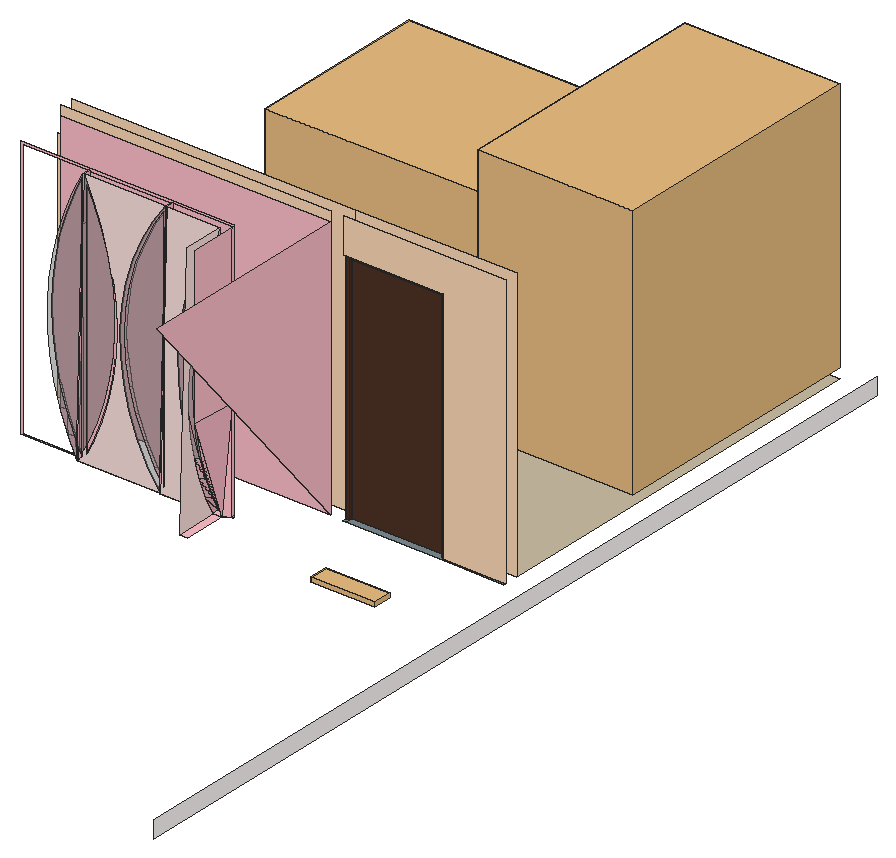
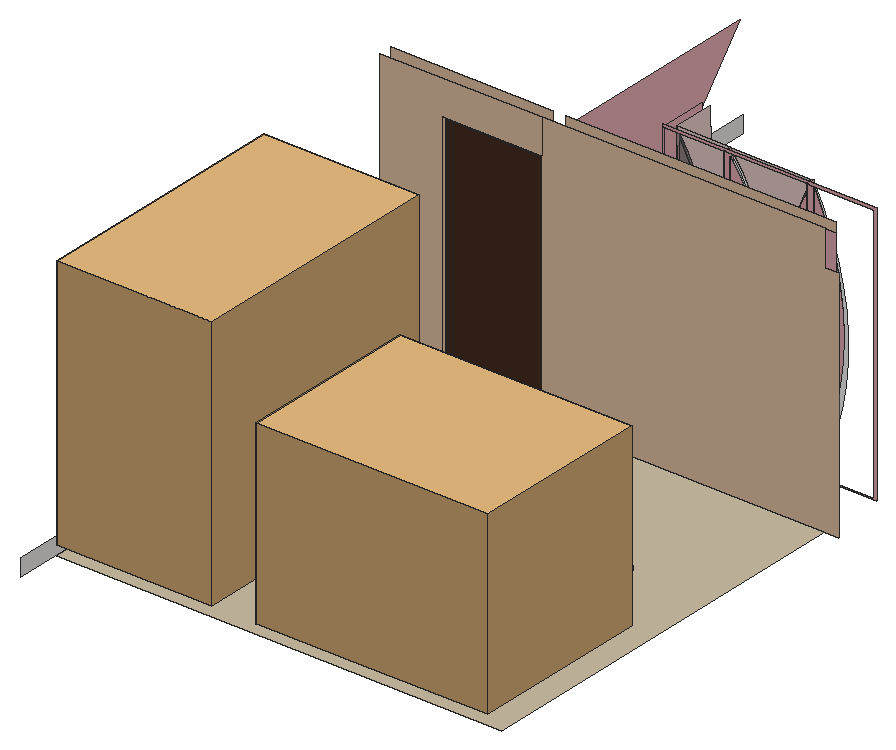
# SketchUp Ruby script. Lengths in inches.
U = 1.inch
M = Sketchup.active_model
def pt(a) = Geom::Point3d.new(a.map { |v| v * U })
def face(e, loops, mat)
  f = e.add_face(loops[0].map { |a| pt(a) })
  loops[1..].each { |l| e.add_face(l.map { |a| pt(a) }).erase! }
  f.material = f.back_material = mat if mat
  f
end
# faces: each face lists its corners as indices into pts; further lists are holes
def faces(e, pts, list, mat = nil) = list.each { |f| face(e, (f[0].is_a?(Array) ? f : [f]).map { |l| l.map { |i| pts[i] } }, mat) }
# xy, xz, yz: faces in a plane at the given z, y or x. An outline is a flat list of corners, or four numbers for a rectangle; further outlines are holes
def ring(l) = l.size == 4 ? [[l[0], l[1]], [l[2], l[1]], [l[2], l[3]], [l[0], l[3]]] : l.each_slice(2).to_a
def flat(e, list, mat, &to3) = list.each { |f| face(e, (f[0].is_a?(Array) ? f : [f]).map { |l| ring(l).map { |u, v| to3.(u, v) } }, mat) }
def xy(e, z, list, mat = nil) = flat(e, list, mat) { |x, y| [x, y, z] }
def xz(e, y, list, mat = nil) = flat(e, list, mat) { |x, z| [x, y, z] }
def yz(e, x, list, mat = nil) = flat(e, list, mat) { |y, z| [x, y, z] }
def lines(e, pts, list) = list.each { |a, b| e.add_line(pt(pts[a]), pt(pts[b])) }
# prism: a flat outline (further loops are holes) pulled along v
def prism(e, loops, v, mat = nil)
  f = face(e, loops, mat); d = Geom::Vector3d.new(v.map { |x| x * U })
  f.pushpull(f.normal.samedirection?(d) ? d.length : -d.length)
end
def box(e, o, s, mat = nil) = prism(e, [[o, [o[0] + s[0], o[1], o[2]], [o[0] + s[0], o[1] + s[1], o[2]], [o[0], o[1] + s[1], o[2]]]], [0, 0, s[2]], mat)
def at(x, y, z, deg = 0) = Geom::Transformation.translation(pt([x, y, z])) * Geom::Transformation.rotation(ORIGIN, Z_AXIS, deg.degrees)
def axes(o, x, y, z) = Geom::Transformation.new([*x, 0, *y, 0, *z, 0, *pt(o).to_a, 1])
def part(name) = M.definitions.add(name)
# library, detail: a bought-in or finely detailed component or shape, given as its bounding box
def library(name, o, s) = part(name).tap { |d| box(d.entities, o, s) }
def detail(e, o, s) = box(e.add_group.entities, o, s)
def put(e, d, t, mat = nil) = e.add_instance(d, t).tap { |i| i.material = mat if mat }
def group(e, t, mat = nil) = e.add_group.tap { |g| g.transformation = t; g.material = mat if mat }.entities
root = M.entities
M.materials.add("Polis06_194").color = [79, 50, 36]
M.materials.add("[0006_Pink]").color = [255, 192, 203]
M.materials.add("[0007_MistyRose]").color = [255, 228, 225]
M.materials.add("[0010_Snow]").color = [255, 250, 250]
M.materials.add("[0027_PeachPuff]").color = [255, 218, 185]
M.materials.add("[0093_AliceBlue]").color = [240, 248, 255]
M.materials.add("[Concrete Pavers Block Multi]").color = [124, 140, 145]
M.materials.add("[Concrete Tile]").color = [203, 190, 164]
M.materials.add("[Translucent Glass Gray]").color = [128, 128, 128]
M.materials["[Translucent Glass Gray]"].alpha = 0.5
c1 = library("Bedroom1",[0.98,0,0],[44.34,8.22,2])
c2 = library("Bed 003",[-38.05,-87.1,0],[75.86,87.1,55.12])
c3 = part("Interior door")
xy(c3.entities,0,[[0,0,4.72,1.18],[0,34.25,4.72,35.43]],"Polis06_194")
xy(c3.entities,85.26,[[0,1.18,4.72,34.25]],"Polis06_194")
xy(c3.entities,86.61,[[0,0,4.72,35.43]],"Polis06_194")
xz(c3.entities,0,[[0,0,4.72,86.61]],"Polis06_194")
xz(c3.entities,1.18,[[0,0,2.36,85.26],[2.36,0,4.72,85.26]],"Polis06_194")
xz(c3.entities,34.25,[[0,0,4.72,85.26]],"Polis06_194")
xz(c3.entities,35.43,[[0,0,4.72,86.61]],"Polis06_194")
yz(c3.entities,0,[[0,0,1.18,86.61],[34.25,0,35.43,86.61],[1.18,85.26,34.25,86.61]],"Polis06_194")
yz(c3.entities,2.36,[[1.18,0,34.25,0,34.25,85.21,1.18,85.26]],"Polis06_194")
yz(c3.entities,4.72,[[0,0,1.18,86.61],[34.25,0,35.43,86.61],[1.18,85.26,34.25,86.61]],"Polis06_194")
c4 = library("wardrobe\#1",[0.19,0,0],[43.3,8.22,2])
c5 = library("toilet 1",[0.13,0,0],[28.4,8.22,2])
xy(root,0,[[490.5625,345.21,492.04,347.21],[492.04,345.21,535.05,348.7],[535.05,345.21,562.5625,345.9375]],"[Concrete Pavers Block Multi]")
xy(root,0,[[492.04,348.7,533.35,350.1875],[490.5625,350.1875,534.83,351.9375],[364.5625,351.9375,562.5625,531.9375]],"[Concrete Tile]")
xy(root,0.5,[[453.1,301.65,453.1,320.15,429.42,320.15,429.42,320.52,456.54,320.52,456.54,301.65],[392.54,320.52,392.64,320.625,394.9375,321.02,394.9375,322.95,395.4375,323.46,431.8125,323.46,428.92,320.52],[429.42,320.52,432.3125,323.46,459.4375,323.46,459.4375,322.46,456.54,320.52],[392.64,320.625,393.03,321.02,394.9375,321.02],[393.03,321.02,394.9375,322.95,394.9375,321.02]],"[0006_Pink]")
xz(root,319.25,[[456,4.09,456.75,112.22]],"[0006_Pink]")
xz(root,320.15,[[454.84,4.76,454.84,69.55,453.28,7.4]],"[0006_Pink]")
xz(root,320.15,[[429.42,0.5,453.1,0.5,448.16,9.39,444.09,18.71,440.95,28.39,438.76,38.32,437.54,48.42,437.3,58.59,438.05,68.73,439.78,78.76,442.46,88.57,446.09,98.07,450.61,107.18,456,115.8125,432.3125,115.8125]],"[0007_MistyRose]")
xz(root,320.15,[[453.1,0.5,453.28,7.4,451.86,9.8,447.61,18.92,444.27,28.4,441.86,38.16,440.4,48.11,439.91,58.16,440.4,68.2,441.86,78.15,444.27,87.91,447.61,97.4,451.86,106.51,454.84,111.56,454.84,69.55,456,115.8125,450.61,107.18,446.09,98.07,442.46,88.57,439.78,78.76,438.05,68.73,437.3,58.59,437.54,48.42,438.76,38.32,440.95,28.39,444.09,18.71,448.16,9.39],[453.28,7.4,454.84,69.55,454.84,111.56,451.86,106.51,447.61,97.4,444.27,87.91,441.86,78.15,440.4,68.2,439.91,58.16,440.4,48.11,441.86,38.16,444.27,28.4,447.61,18.92,451.86,9.8]],"[Translucent Glass Gray]")
xz(root,320.52,[[392.54,0.5,394.09,3.36,392.6875,6.28],[394.45,2.62,394.45,4.02,394.09,3.36],[396.41,4.55,399.12,9.85,402.875,19.08,405.82,28.59,407.94,38.33,409.22,48.2,409.65,58.16,409.22,68.11,407.94,77.99,407.79,78.69,407.96,77.82,409,67.82,409.18,57.77,408.49,47.75,406.95,37.82,404.57,28.06,401.35,18.54,397.34,9.33,396.41,7.63]],"[0006_Pink]")
xz(root,320.52,[[392.54,0.5,428.92,0.5,423.43,9.21,418.9,18.46,415.38,28.14,412.92,38.14,411.53,48.34,411.24,58.64,412.05,68.9,413.94,79.02,416.91,88.89,420.91,98.375,425.89,107.39,431.8125,115.8125,395.4375,115.8125,399.78,106.75,403.33,97.35,406.07,87.68,407.79,78.69,407.94,77.99,409.22,68.11,409.65,58.16,409.22,48.2,407.94,38.33,405.82,28.59,402.875,19.08,399.12,9.85,396.41,4.55,396.41,7.63,394.45,4.02,394.45,2.62,394.09,3.36]],"[0007_MistyRose]")
xz(root,320.52,[[392.04,0.5,392.21,7.26,391.03,9.7,387.45,19,384.63,28.56,382.61,38.3125,381.39,48.2,380.98,58.16,381.39,68.11,382.61,78,384.63,87.76,387.45,97.31,391.03,106.61,394.45,113.69,394.45,96.52,394.9375,115.8125,390.36,106.91,386.53,97.67,383.46,88.14,381.1875,78.4,379.71,68.5,379.05,58.52,379.21,48.51,380.18,38.55,381.97,28.71,384.55,19.04,387.92,9.62],[428.92,0.5,429.06,6.18,426.85,9.51,422.13,18.55,418.41,28.05,415.71,37.89,414.09,47.97,413.54,58.16,414.09,68.35,415.71,78.42,418.41,88.26,422.13,97.76,426.85,106.81,430.96,112.99,430.96,81.8125,431.8125,115.8125,425.89,107.39,420.91,98.375,416.91,88.89,413.94,79.02,412.05,68.9,411.24,58.64,411.53,48.34,412.92,38.14,415.38,28.14,418.9,18.46,423.43,9.21],[394.09,3.36,394.45,4.02,394.45,76.61,392.6875,6.28],[394.45,4.02,396.41,7.63,396.41,111.77,399.12,106.46,402.875,97.23,405.82,87.72,407.79,78.69,406.07,87.68,403.33,97.35,399.78,106.75,395.4375,115.8125,394.45,76.61],[429.06,6.18,430.96,81.8125,430.96,112.99,426.85,106.81,422.13,97.76,418.41,88.26,415.71,78.42,414.09,68.35,413.54,58.16,414.09,47.97,415.71,37.89,418.41,28.05,422.13,18.55,426.85,9.51],
  [392.21,7.26,394.45,96.52,394.45,113.69,391.03,106.61,387.45,97.31,384.63,87.76,382.61,78,381.39,68.11,380.98,58.16,381.39,48.2,382.61,38.3125,384.63,28.56,387.45,19,391.03,9.7],[396.41,7.63,397.34,9.33,401.35,18.54,404.57,28.06,406.95,37.82,408.49,47.75,409.18,57.77,409,67.82,407.96,77.82,407.79,78.69,405.82,87.72,402.875,97.23,399.12,106.46,396.41,111.77]],"[Translucent Glass Gray]")
xz(root,320.9,[[396.41,4.55,399.12,9.85,402.875,19.08,405.82,28.59,407.94,38.33,409.22,48.2,409.65,58.16,409.22,68.11,407.94,77.99,405.82,87.72,402.875,97.23,399.12,106.46,396.41,111.77]],"[0006_Pink]")
xz(root,321.02,[[394.45,2.62,394.45,113.69,391.03,106.61,387.45,97.31,384.63,87.76,382.61,78,381.39,68.11,380.98,58.16,381.39,48.2,382.61,38.3125,384.63,28.56,387.45,19,391.03,9.7]],"[0006_Pink]")
xz(root,321.71,[[430.96,3.32,430.96,112.99,426.85,106.81,422.13,97.76,418.41,88.26,415.71,78.42,414.09,68.35,413.54,58.16,414.09,47.97,415.71,37.89,418.41,28.05,422.13,18.55,426.85,9.51]],"[0006_Pink]")
xz(root,323.46,[[[364.5625,0,459.4375,0,459.4375,0.5,432.3125,0.5,432.3125,115.8125,459.4375,115.8125,459.4375,116.8125,364.5625,116.8125],[395.4375,0.5,431.8125,115.8125],[365.5625,0.5,394.9375,115.8125]]],"[0006_Pink]")
xz(root,345.9375,[[364.5625,0,484.5625,116.8125]],"[0006_Pink]")
xz(root,345.9375,[[364.5625,0,484.5625,121.1875],[534.83,0,562.5625,0,562.5625,121.1875,490.5625,121.1875,490.5625,105.875,534.83,105.875]],"[0027_PeachPuff]")
xz(root,351.9375,[[358.5625,0,358.5625,105.53,364.5625,105.53,364.5625,121.1875,490.5625,121.1875,490.5625,0],[534.83,0,534.83,105.875,490.5625,105.875,490.5625,121.1875,562.5625,121.1875,562.5625,0]],"[0027_PeachPuff]")
yz(root,394.45,[[320.52,2.62,321.02,113.69]],"[0006_Pink]")
yz(root,394.9375,[[321.02,0.5,323.46,0.5,323.46,115.8125,320.52,115.8125]],"[0006_Pink]")
yz(root,396.41,[[320.52,4.55,320.9,111.77]],"[0006_Pink]")
yz(root,430.96,[[320.52,3.32,321.71,112.99]],"[0006_Pink]")
yz(root,431.8125,[[323.46,0.5,323.46,115.8125,320.52,115.8125]],"[0006_Pink]")
yz(root,456,[[319.25,4.09,316.19,9.78,312.27,18.98,309.18,28.5,306.96,38.25,305.625,48.16,305.18,58.16,305.625,68.15,306.96,78.0625,309.18,87.82,312.27,97.33,316.19,106.54,319.25,112.22]],"[Translucent Glass Gray]")
yz(root,456.75,[[319.25,4.09,319.25,112.22,316.19,106.54,312.27,97.33,309.18,87.82,306.96,78.0625,305.625,68.15,305.18,58.16,305.625,48.16,306.96,38.25,309.18,28.5,312.27,18.98,316.19,9.78]],"[0006_Pink]")
yz(root,459.4375,[[323.46,0,322.46,0.5,323.46,0.5],[322.46,0.5,322.46,45.68,323.46,45.625,323.46,0.5],[323.46,45.625,322.46,45.68,322.46,115.8125,323.46,115.8125],[322.46,45.68,322.46,115.8125,301.71,115.8125,301.71,46.85]],"[0006_Pink]")
yz(root,484.5625,[[345.9375,0,345.9375,116.8125,249.21,116.8125]],"[0006_Pink]")
yz(root,534.83,[[345.9375,0,351.9375,105.875]],"[0027_PeachPuff]")
yz(root,571.5625,[[138.9375,-7.5625,540.9375,0]],"[0010_Snow]")
p = [[459.4375,322.46,0.5],[459.4375,323.46,0],[456.54,320.52,0.5],[453.1,320.15,0.5],[453.1,301.65,0.5],[456,301.65,115.8125],
  [456,320.15,115.8125],[455.78,315.38,106.93],[455.54,311.42,97.65],[455.3,308.31,88.06],[455.06,306.07,78.22],[454.81,304.72,68.23],
  [454.55,304.27,58.16],[454.3,304.72,48.08],[454.05,306.07,38.09],[453.8,308.31,28.26],[453.56,311.42,18.66],[453.33,315.38,9.39],
  [459.4375,322.46,45.68],[459.4375,301.71,46.85],[456,319.25,4.09],[454.84,320.15,69.55],[453.28,320.15,7.4],[456,319.25,112.22],
  [432.3125,320.15,115.8125],[432.3125,323.46,115.8125],[429.42,320.52,0.5],[429.42,320.15,0.5],[387.92,320.52,9.62],[390.59,321.02,9.51],
  [392.04,320.52,0.5],[394.9375,321.02,0.5],[392.64,320.625,0.5],[394.9375,320.52,115.8125],[394.45,320.52,96.52],[392.21,320.52,7.26],
  [395.4375,323.46,0.5],[394.9375,322.95,0.5],[393.03,321.02,0.5],[392.54,320.52,0.5],[395.4375,323.46,115.8125],[395.4375,320.52,115.8125],
  [392.6875,320.52,6.28],[394.45,320.52,76.61],[428.92,320.52,0.5],[431.8125,323.46,0.5],[431.8125,320.52,115.8125],[430.96,320.52,81.8125],
  [429.06,320.52,6.18],[432.3125,323.46,0.5],[394.45,321.02,2.62],[391.03,321.02,9.7],[391.03,320.52,9.7],[394.09,320.52,3.36],
  [394.45,320.52,2.62],[426.85,320.52,9.51],[430.96,320.52,3.32],[430.96,321.71,3.32],[426.85,321.71,9.51],[456,316.19,9.78],
  [456.75,316.19,9.78],[456.75,319.25,4.09],[396.41,320.52,4.55],[399.12,320.52,9.85],[399.12,320.9,9.85],[396.41,320.9,4.55],
  [386.99,321.02,18.84],[422.13,320.52,18.55],[422.13,321.71,18.55],[384.55,320.52,19.04],[387.45,321.02,19],[387.45,320.52,19],
  [456,312.27,18.98],[456.75,312.27,18.98],[402.875,320.52,19.08],[402.875,320.9,19.08],[418.41,320.52,28.05],[418.41,321.71,28.05],
  [456,309.18,28.5],[456.75,309.18,28.5],[384.63,321.02,28.56],[384.63,320.52,28.56],[405.82,320.52,28.59],[405.82,320.9,28.59],
  [415.71,320.52,37.89],[415.71,321.71,37.89],[407.94,320.52,38.33],[407.94,320.9,38.33],[414.09,320.52,47.97],[414.09,321.71,47.97],
  [409.22,320.52,48.2],[409.22,320.9,48.2]]
faces(root,p,[[0,1,2],[18,19,2],[3,17,20],[6,21,22,3,23],[24,25,26,27],[28,29,30],[31,32,30,29],[32,31,33,34,35,30],
  [36,37,38,32,39,40],[41,40,39,42,43],[44,45,46,47,48],[49,26,25],[0,18,2],[50,51,52,35,42,53,54],[55,48,56,57,58],[59,20,17],
  [60,59,20,61],[62,63,64,65],[17,16,59],[29,28,66],[67,55,58,68],[69,66,28],[51,70,71,52],[72,59,16],
  [73,72,59,60],[63,74,75,64],[76,67,68,77],[16,15,72],[78,72,15],[79,78,72,73],[70,80,81,71],[74,82,83,75],
  [84,76,77,85],[82,86,87,83],[88,84,85,89],[86,90,91,87]],"[0006_Pink]")
faces(root,p,[[3,4,5,6,7,8,9,10,11,12,13,14,15,16,17]],"[0007_MistyRose]")
faces(root,p,[[20,23,3]],"[Translucent Glass Gray]")
detail(root,[493.45,416.65,4.375],[69.11,115.29,113.3])
put(root,c1,at(398.39,415.33,0))
put(root,c2,axes([427.22,526.02,0],[1.3566,0,0],[0,0.92,0],[0,0,1.449]),"[0093_AliceBlue]")
put(root,c3,axes([490.5625,350.1875,0],[0,-0.63,0],[1.24934,0,0],[0,0,1.22238]),"[0006_Pink]")
put(root,c4,at(499.46,479.17,0))
put(root,c5,at(509.07,304.53,0))
